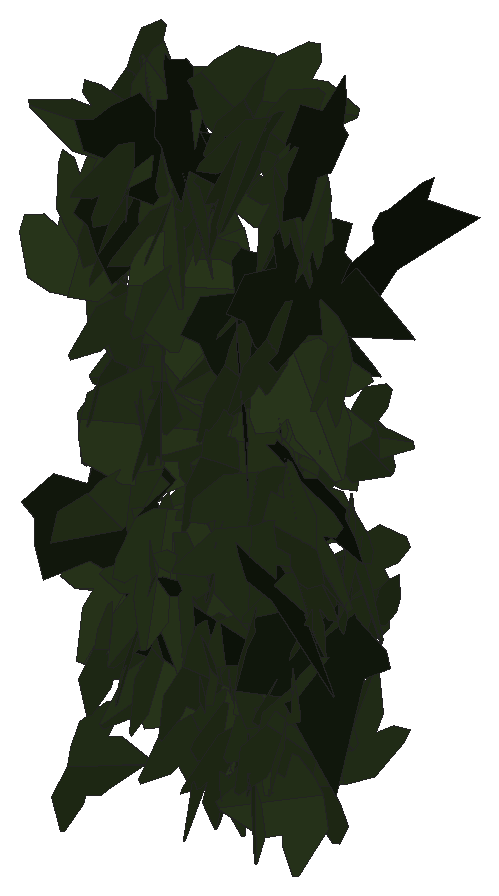
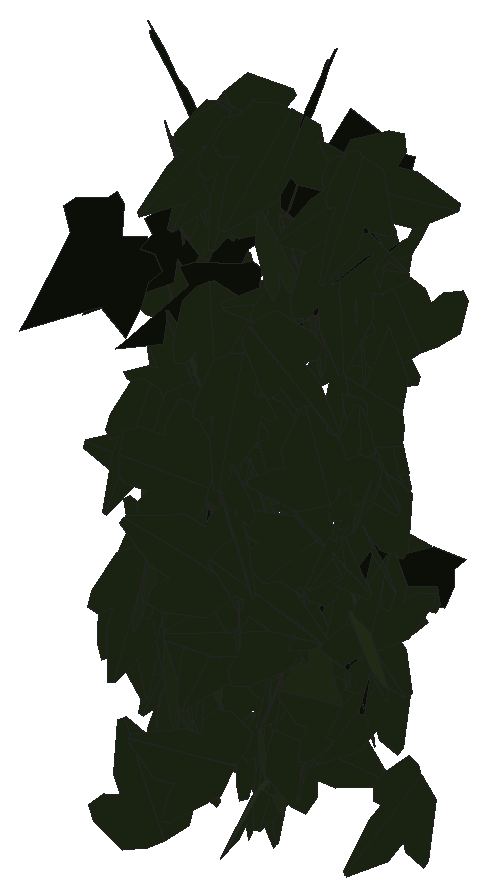
# SketchUp Ruby script. Lengths in inches.
U = 1.inch
M = Sketchup.active_model
def pt(a) = Geom::Point3d.new(a.map { |v| v * U })
def face(e, loops, mat)
  f = e.add_face(loops[0].map { |a| pt(a) })
  loops[1..].each { |l| e.add_face(l.map { |a| pt(a) }).erase! }
  f.material = f.back_material = mat if mat
  f
end
# faces: each face lists its corners as indices into pts; further lists are holes
def faces(e, pts, list, mat = nil) = list.each { |f| face(e, (f[0].is_a?(Array) ? f : [f]).map { |l| l.map { |i| pts[i] } }, mat) }
# xy, xz, yz: faces in a plane at the given z, y or x. An outline is a flat list of corners, or four numbers for a rectangle; further outlines are holes
def ring(l) = l.size == 4 ? [[l[0], l[1]], [l[2], l[1]], [l[2], l[3]], [l[0], l[3]]] : l.each_slice(2).to_a
def flat(e, list, mat, &to3) = list.each { |f| face(e, (f[0].is_a?(Array) ? f : [f]).map { |l| ring(l).map { |u, v| to3.(u, v) } }, mat) }
def xy(e, z, list, mat = nil) = flat(e, list, mat) { |x, y| [x, y, z] }
def xz(e, y, list, mat = nil) = flat(e, list, mat) { |x, z| [x, y, z] }
def yz(e, x, list, mat = nil) = flat(e, list, mat) { |y, z| [x, y, z] }
def lines(e, pts, list) = list.each { |a, b| e.add_line(pt(pts[a]), pt(pts[b])) }
# prism: a flat outline (further loops are holes) pulled along v
def prism(e, loops, v, mat = nil)
  f = face(e, loops, mat); d = Geom::Vector3d.new(v.map { |x| x * U })
  f.pushpull(f.normal.samedirection?(d) ? d.length : -d.length)
end
def box(e, o, s, mat = nil) = prism(e, [[o, [o[0] + s[0], o[1], o[2]], [o[0] + s[0], o[1] + s[1], o[2]], [o[0], o[1] + s[1], o[2]]]], [0, 0, s[2]], mat)
def at(x, y, z, deg = 0) = Geom::Transformation.translation(pt([x, y, z])) * Geom::Transformation.rotation(ORIGIN, Z_AXIS, deg.degrees)
def axes(o, x, y, z) = Geom::Transformation.new([*x, 0, *y, 0, *z, 0, *pt(o).to_a, 1])
def part(name) = M.definitions.add(name)
# library, detail: a bought-in or finely detailed component or shape, given as its bounding box
def library(name, o, s) = part(name).tap { |d| box(d.entities, o, s) }
def detail(e, o, s) = box(e.add_group.entities, o, s)
def put(e, d, t, mat = nil) = e.add_instance(d, t).tap { |i| i.material = mat if mat }
def group(e, t, mat = nil) = e.add_group.tap { |g| g.transformation = t; g.material = mat if mat }.entities
root = M.entities
M.materials.add("efeu1").color = [18, 25, 13]
M.materials.add("efeu2").color = [43, 57, 29]
c1 = part("ivyleaf_10")
p = [[0,0.5,-0.03],[-0.0625,2.02,-0.43],[-0.19,2.01,-0.46],[-0.54,1.05,-0.29],[-0.52,0.625,-0.18],[-0.83,0.76,-0.28],
  [-1.16,0.64,-0.33],[-1.15,0.33,-0.24],[-0.77,-0.39,0.02],[-0.3,-0.51,0.16],[0.04,-0.48,0.23],[-0.02,2.01,-0.4375],
  [-0.06,2.01,-0.43],[0.04,-0.49,0.23],[0.67,-0.49,0.14],[1.38,0.36,-0.2],[1.375,0.51,-0.24],[0.81,0.65,-0.19],
  [0.62,0.59,-0.15],[0.6,1.09,-0.28],[0.5,1.23,-0.31]]
faces(c1.entities,p,[[0,1,2,3,4,5,6,7,8,9,10],[11,12,0,13,14,15,16,17,18,19,20]],"efeu2")
c2 = part("ivyleaf_9")
p = [[1.54,2.16,1.25],[1.36,2.04,1.19],[-0.21,0.99,0.68],[-0.71,1.11,0.82],[-0.85,0.86,0.67],[-0.8,0.17,0.21],
  [-0.9,-0.01,0.1],[-0.67,-0.16,-0.02],[-0.08,-0.08,-0.05],[-0.03,-0.6,-0.4],[0.65,-0.88,-0.66],[0.83,-0.6,-0.49],
  [1.29,-0.42,-0.43],[1.8125,-0.07,-0.26],[1.21,0.44,0.15]]
faces(c2.entities,p,[[0,1,2,3,4,5,6,7,8,9,10,11,12,13,14]],"efeu1")
put(root,c1,axes([17.64,224.54,212.18],[0.2615,0.37788,-0.19704],[0.11551,0.15967,0.45952],[0.41021,-0.28585,-0.00379]))
put(root,c1,axes([17.67,225.08,210.66],[-0.06959,-0.33909,-0.3608],[0.20664,0.31121,-0.33234],[0.44995,-0.19537,0.09683]))
put(root,c1,axes([18.18,224.62,213.66],[-0.00757,0.03788,-0.49851],[-0.49654,0.0575,0.01191],[0.05823,0.49524,0.03675]))
put(root,c1,axes([17.86,224.87,209.08],[0.13792,0.47951,-0.03238],[-0.01347,0.03753,0.49841],[0.48041,-0.13661,0.02327]))
put(root,c1,axes([17.9,224.31,212.84],[0.04507,0.18765,-0.46125],[-0.0477,0.46264,0.18355],[0.49567,0.02745,0.0596]))
put(root,c1,axes([17.85,225.125,214.01],[-0.01418,-0.36054,-0.34613],[0.03369,0.3448,-0.36053],[0.49866,-0.03355,0.01451]))
put(root,c1,axes([17.9,225.35,213.2],[-0.1867,-0.46323,-0.0237],[0.00829,0.02221,-0.49944],[0.46376,-0.18688,-0.00061]))
put(root,c1,axes([17.83,224.4,207.17],[-0.04942,-0.21754,-0.44748],[0.10686,0.43454,-0.22305],[0.48594,-0.11768,0.00354]))
put(root,c1,axes([17.92,224.92,211.2],[-0.00617,-0.38233,-0.32216],[0.02352,0.32161,-0.38212],[0.49941,-0.01988,0.01402]))
put(root,c1,axes([18.3,224.91,211.08],[-0.17671,0.01361,0.46753],[-0.46773,-0.00286,-0.1767],[-0.00213,-0.49981,0.01374]))
put(root,c1,axes([17.75,225.18,211.18],[-0.20677,0.25144,-0.3795],[0.21731,-0.31174,-0.32495],[-0.40003,-0.29932,0.01963]))
put(root,c1,axes([17.87,225.59,210.96],[0.41138,0.26596,-0.10014],[0.08042,0.06005,0.48982],[0.27257,-0.41912,0.00663]))
put(root,c1,axes([17.71,225.07,208.91],[0.15502,-0.28412,-0.38111],[0.25032,-0.29199,0.3195],[-0.40411,-0.28986,0.05172]))
put(root,c1,axes([17.6,224.98,211.71],[-0.009,-0.05461,0.49693],[0.49966,-0.01693,0.00719],[0.01604,0.49672,0.05487]))
put(root,c2,axes([17.74,224.67,209.85],[0.01818,-0.30174,-0.39827],[0.13086,0.3875,-0.28761],[0.48223,-0.09378,0.09306]))
put(root,c1,axes([18.375,225.36,210.3],[-0.15751,-0.00285,0.47453],[-0.47294,-0.04009,-0.15722],[0.03894,-0.49838,0.00994]))
put(root,c1,axes([17.93,224.59,209.79],[-0.26802,-0.31765,-0.27796],[0.18909,0.20402,-0.41548],[0.37737,-0.32783,0.01077]))
put(root,c1,axes([18.04,224.74,212.79],[0.14301,-0.45229,-0.15806],[0.00861,0.16735,-0.47108],[0.47904,0.13201,0.05565]))
put(root,c1,axes([18.01,224.57,208.37],[-0.05576,-0.22516,-0.44294],[0.12172,0.42595,-0.23184],[0.48174,-0.13369,0.00731]))
put(root,c1,axes([17.74,224.99,209.85],[0.17654,-0.18081,-0.43144],[0.35353,-0.25042,0.24961],[-0.30635,-0.39319,0.03942]))
put(root,c1,axes([18.12,225.3,208.45],[0.18317,-0.24827,0.39346],[-0.16256,0.36205,0.30413],[-0.43592,-0.23933,0.05192]))
put(root,c1,axes([18.18,224.78,209.125],[0.4167,0.1887,-0.20188],[-0.18238,-0.08662,-0.45742],[-0.2076,0.45485,-0.00336]))
put(root,c1,axes([18.1,225.01,213.71],[-0.01135,-0.02598,-0.4992],[0.10029,0.48905,-0.02773],[0.48971,-0.10075,-0.00589]))
put(root,c1,axes([18.21,224.6875,213.42],[-0.00699,-0.48951,0.10164],[-0.00529,-0.10158,-0.48955],[0.49992,-0.00792,-0.00376]))
put(root,c2,axes([17.97,224.84,212.95],[0.26335,-0.29587,-0.30514],[-0.06558,0.32638,-0.37306],[0.41994,0.23651,0.1331]))
put(root,c1,axes([18.34,225.4,208],[-0.08271,-0.24704,0.42677],[-0.13867,-0.40361,-0.26051],[0.47321,-0.16145,-0.00174]))
put(root,c1,axes([18.21,224.68,211.92],[-0.18902,-0.43193,-0.16645],[0.0723,0.15004,-0.47144],[0.45721,-0.20229,0.00574]))
put(root,c1,axes([18.45,225.67,212.3],[0.29862,-0.09169,-0.39041],[-0.36462,0.14058,-0.31191],[0.16697,0.47099,0.0171]))
put(root,c1,axes([17.98,224.65,210.61],[0.07656,0.02642,0.4934],[0.23997,0.43446,-0.06049],[-0.43192,0.24606,0.05384]))
put(root,c1,axes([18.26,224.75,208.76],[0.28808,-0.40856,0.00918],[0.0027,-0.00933,-0.49991],[0.40866,0.28808,-0.00317]))
put(root,c1,axes([18.39,225.13,212.92],[0.15823,-0.46021,-0.11477],[-0.02025,0.11433,-0.48633],[0.47387,0.15855,0.01754]))
put(root,c1,axes([18.35,224.85,208.25],[0.07269,-0.37831,-0.31875],[0.06106,0.32657,-0.37367],[0.49091,0.0154,0.09367]))
put(root,c1,axes([18.43,224.88,212.78],[0.02384,-0.49721,0.04705],[0.0081,-0.04671,-0.49775],[0.49937,0.02449,0.00583]))
put(root,c1,axes([18.47,224.72,209.29],[-0.00281,-0.06953,-0.49513],[-0.02373,0.4946,-0.06932],[0.49943,0.02311,-0.00607]))
put(root,c1,axes([18.11,225.64,210.22],[0.32577,0.15564,0.3459],[0.29949,0.17425,-0.36047],[-0.23276,0.44205,0.0203]))
put(root,c1,axes([18.61,224.71,213.53],[0.34857,-0.09713,0.34506],[-0.33231,0.09292,0.36185],[-0.13442,-0.48159,0.00022]))
put(root,c1,axes([18.61,224.8125,209.14],[-0.16539,-0.36754,0.29591],[-0.11529,-0.27258,-0.403],[0.45755,-0.20154,0.00541]))
put(root,c1,axes([18.77,225.79,209.82],[0.26204,0.02235,-0.42525],[-0.42583,0.01467,-0.26163],[0.00078,0.49929,0.02672]))
put(root,c1,axes([18.56,224.59,211.07],[0.1821,-0.41178,-0.21743],[-0.02812,0.22332,-0.44647],[0.46481,0.17483,0.05818]))
put(root,c1,axes([18.89,224.78,208.43],[-0.07457,0.08537,-0.48698],[-0.40707,0.26891,0.10948],[0.2806,0.4128,0.02939]))
put(root,c1,axes([18.64,225.09,213.11],[0.3578,-0.30703,-0.16647],[-0.12497,0.11,-0.47147],[0.32613,0.37899,0.00198]))
put(root,c2,axes([18.17,224.59,213.44],[0.17994,0.00908,0.46641],[0.46649,-0.00108,-0.17996],[-0.00226,0.49992,-0.00886]))
put(root,c1,axes([18.57,224.71,209.62],[0.16219,0.45037,-0.14443],[-0.0584,-0.13245,-0.47859],[-0.46934,0.17212,0.00964]))
put(root,c1,axes([18.65,225.32,207.62],[-0.43569,0.11451,0.21693],[0.20765,-0.06322,0.45043],[0.13058,0.48259,0.00753]))
put(root,c1,axes([18.87,224.85,208.44],[0.10057,-0.0306,-0.48882],[-0.0991,0.48743,-0.05091],[0.47965,0.10712,0.09198]))
put(root,c2,axes([18.35,224.74,208.71],[0.22121,0.1206,-0.43188],[0.35154,0.25232,0.25052],[0.27837,-0.41448,0.02684]))
put(root,c1,axes([18.54,224.77,213.14],[0.37885,-0.18247,0.27052],[0.26742,-0.06391,-0.41761],[0.18698,0.46111,0.04917]))
put(root,c1,axes([18.71,224.8,212.35],[-0.18406,-0.38631,-0.25862],[0.16046,0.20826,-0.4253],[0.43632,-0.23956,0.04731]))
put(root,c1,axes([19.01,225.35,209.6],[0.34956,0.00602,0.35745],[-0.35547,0.05909,0.34663],[-0.03807,-0.49646,0.04559]))
put(root,c1,axes([18.79,225.2,213.23],[0.1265,-0.44392,0.19219],[0.05226,-0.18495,-0.46159],[0.4809,0.13687,-0.00039]))
put(root,c1,axes([19.1,225.02,208.37],[-0.40068,-0.01049,0.2989],[-0.29853,-0.01653,-0.40076],[0.01829,-0.49962,0.00698]))
put(root,c1,axes([18.63,224.7,209.39],[0.43192,-0.11056,0.22632],[0.22546,-0.0306,-0.44523],[0.1123,0.48666,0.02341]))
put(root,c1,axes([18.78,225.16,214.21],[-0.26561,-0.32596,-0.27056],[0.16918,0.21115,-0.42047],[0.38837,-0.31491,-0.00187]))
put(root,c1,axes([18.99,225.67,210.57],[0.31068,-0.25282,-0.29926],[-0.19872,0.22745,-0.39847],[0.33762,0.36653,0.04085]))
put(root,c1,axes([18.61,224.95,208.16],[0.39618,0.16741,0.25498],[0.22652,0.11843,-0.42972],[-0.20427,0.45601,0.01799]))
put(root,c1,axes([18.5625,224.61,212.3125],[-0.0135,-0.0784,-0.49363],[0.44217,0.22836,-0.04836],[0.23304,-0.43784,0.06316]))
put(root,c1,axes([18.88,224.8,207.73],[-0.19827,-0.40639,-0.21339],[0.09689,0.19016,-0.45216],[0.44867,-0.22065,0.00335]))
put(root,c2,axes([18.9,224.38,214.39],[0.26883,-0.15755,-0.39104],[-0.3176,0.22931,-0.31073],[0.27724,0.41545,0.02322]))
put(root,c1,axes([18.96,225.5,211.67],[-0.12469,-0.44761,-0.18465],[0.05343,0.17679,-0.46464],[0.48125,-0.1356,0.00375]))
put(root,c1,axes([18.96,225.09,207.28],[0.22271,-0.13905,-0.42552],[0.00503,0.47602,-0.15292],[0.44763,0.06383,0.21343]))
put(root,c1,axes([18.75,225.26,208.99],[0.02995,-0.08089,0.4925],[0.25836,0.42465,0.05404],[-0.42703,0.25125,0.06724]))
put(root,c1,axes([19.03,224.49,208.53],[-0.02806,-0.32135,-0.38203],[0.04211,0.37974,-0.32252],[0.49743,-0.05027,0.00575]))
put(root,c1,axes([19.06,225.32,211.47],[-0.04127,0.0057,-0.49826],[-0.12243,-0.48476,0.0046],[-0.48302,0.12238,0.04141]))
put(root,c1,axes([19,224.5,213.62],[-0.2848,0.41096,0.00067],[-0.00041,0.00053,-0.5],[-0.41096,-0.2848,0.00004]))
put(root,c1,axes([18.95,225.02,207.61],[0.18206,-0.3612,0.29392],[0.13835,-0.25938,-0.40445],[0.44465,0.2286,0.00551]))
put(root,c1,axes([19.11,225.02,207.58],[0.04931,-0.49739,-0.01299],[-0.00089,0.01296,-0.49983],[0.49756,0.04931,0.00039]))
put(root,c1,axes([19.05,225.19,211.21],[0.49808,-0.03349,-0.02821],[-0.02746,0.01204,-0.4991],[0.03411,0.49873,0.01015]))
put(root,c1,axes([18.92,225.91,207.82],[0.14371,0.17618,-0.44532],[0.27391,0.35114,0.22731],[0.39284,-0.30929,0.00441]))
put(root,c1,axes([19.12,225.23,214.02],[-0.11242,-0.42007,-0.24678],[0.06639,0.23769,-0.43485],[0.48265,-0.13054,0.00233]))
put(root,c1,axes([19.36,225.12,209.625],[-0.23062,0.18756,0.40204],[-0.34545,0.20837,-0.29537],[-0.27835,-0.41401,0.03348]))
put(root,c1,axes([19.14,224.92,210.16],[0.29836,-0.39089,0.0905],[0.06199,-0.06651,-0.49166],[0.39641,0.30461,0.00878]))
put(root,c1,axes([19,225.84,209.77],[-0.09889,-0.32395,0.3678],[0.21446,0.30878,0.32964],[-0.44071,0.22296,0.07788]))
put(root,c1,axes([19.68,224.97,210.52],[-0.08826,-0.03157,0.49113],[-0.47837,-0.11173,-0.09315],[0.11563,-0.48633,-0.01048]))
put(root,c1,axes([19.36,224.32,210.91],[0.0193,-0.29949,-0.39992],[0.01876,0.40037,-0.29892],[0.49928,-0.00347,0.02669]))
put(root,c1,axes([19.34,224.8125,213.81],[0.19916,-0.45166,0.07962],[0.02181,-0.07737,-0.4935],[0.45811,0.20004,-0.01111]))
put(root,c1,axes([19.5,225.34,211.1],[-0.47127,-0.06799,0.15258],[-0.14825,-0.0402,-0.47582],[0.07697,-0.49372,0.01773]))
put(root,c1,axes([19.41,225.34,212.2],[-0.0938,-0.48863,-0.04944],[0.00668,0.04906,-0.49754],[0.49108,-0.094,-0.00267]))
put(root,c1,axes([19.3,225.4375,214.09],[-0.02435,-0.24474,-0.43533],[0.19696,0.39581,-0.23354],[0.45893,-0.18285,0.07714]))
put(root,c1,axes([19.78,225.17,213.3],[0.06918,0.05139,-0.49252],[-0.49302,0.05364,-0.06366],[0.0463,0.49445,0.0581]))
put(root,c1,axes([19.5,224.87,214.03],[0.00975,-0.482,0.13259],[-0.01053,-0.13278,-0.48193],[0.49979,0.0066,-0.01274]))
put(root,c1,axes([19.39,225.08,208.875],[-0.32792,-0.3004,-0.22854],[0.16211,0.16132,-0.44463],[0.34087,-0.3657,-0.0084]))
put(root,c1,axes([19.48,224.5,211.78],[-0.00525,-0.34804,-0.35894],[0.02788,0.3582,-0.34773],[0.49919,-0.02367,0.01564]))
put(root,c1,axes([19.14,225.26,209.98],[0.09245,0.06472,0.4871],[0.3698,0.31722,-0.11233],[-0.32357,0.38103,0.01079]))
put(root,c1,axes([19.47,225.12,213.97],[-0.14401,-0.35418,-0.32221],[0.11517,0.30097,-0.3823],[0.46476,-0.18433,-0.0051]))
put(root,c1,axes([19.72,224.46,208.65],[-0.00398,-0.0129,0.49982],[-0.30944,0.39267,0.00767],[-0.39272,-0.30927,-0.01111]))
put(root,c2,axes([19.26,224.9375,212.26],[0.13956,-0.14688,-0.45711],[0.15377,0.46463,-0.10235],[0.45484,-0.11201,0.17486]))
put(root,c1,axes([19.65,224.62,210.54],[-0.22268,-0.44581,0.04087],[-0.01627,-0.03756,-0.49832],[0.44738,-0.22326,0.00222]))
put(root,c1,axes([19.66,224.57,210.01],[-0.29602,-0.40285,-0.00924],[0.00734,0.00607,-0.49991],[0.40289,-0.2961,0.00232]))
put(root,c1,axes([19.48,224.93,207.64],[-0.11139,0.39312,-0.28818],[0.082,-0.27628,-0.40859],[-0.48049,-0.13828,-0.00292]))
put(root,c2,axes([19.34,224.83,211.68],[0.01373,-0.02945,-0.49894],[0.47694,-0.14848,0.02189],[-0.14946,-0.47654,0.02402]))
put(root,c2,axes([19.83,224.86,210.82],[0.1669,-0.00507,-0.47129],[-0.46063,0.10413,-0.16425],[0.09982,0.48901,0.03009]))
put(root,c1,axes([19.59,226.01,207.06],[-0.1308,-0.47786,0.06737],[0.02066,0.06419,0.49543],[-0.48215,0.13239,0.00295]))
put(root,c1,axes([19.72,225.22,213.58],[0.06066,-0.43727,0.23476],[0.05507,-0.22912,-0.44099],[0.49324,0.07936,0.02037]))
put(root,c1,axes([20.07,224.75,207.4375],[0.22366,-0.06155,-0.44293],[-0.42761,0.1155,-0.23197],[0.13087,0.48257,-0.00097]))
put(root,c1,axes([19.67,225.58,208.49],[0.17487,-0.40721,0.23152],[0.16765,-0.17635,-0.4368],[0.43739,0.23039,0.07486]))
put(root,c1,axes([19.44,225.72,210.57],[-0.05154,-0.14036,0.47712],[0.4402,0.21036,0.10944],[-0.23145,0.43133,0.10189]))
put(root,c1,axes([19.77,225,213.6],[-0.16491,0.47179,0.01478],[-0.00673,0.0133,-0.49978],[-0.47197,-0.16504,0.00196]))
put(root,c1,axes([20.16,225.03,207.47],[-0.1996,0.0465,0.45607],[-0.45079,0.07052,-0.20448],[-0.08334,-0.49281,0.01377]))
put(root,c1,axes([19.77,224.9,208.4],[0.21095,-0.40624,0.20118],[0.07945,-0.18533,-0.45754],[0.44631,0.225,-0.01364]))
put(root,c1,axes([19.84,225.27,207.82],[0.06131,-0.46586,0.17093],[0.01997,-0.16977,-0.46987],[0.49582,0.06445,-0.00221]))
put(root,c1,axes([19.89,224.58,212.14],[-0.0473,-0.38855,-0.31112],[0.02292,0.31049,-0.39124],[0.49723,-0.05127,-0.01156]))
put(root,c1,axes([19.72,224.82,208.48],[0.43307,-0.18471,0.16833],[0.15796,-0.05865,-0.47075],[0.19365,0.46092,0.00756]))
put(root,c1,axes([19.95,225.13,209.45],[-0.17221,-0.46935,-0.0076],[0.0034,0.00685,-0.49994],[0.4694,-0.17224,0.00083]))
put(root,c1,axes([19.83,224.82,208.17],[-0.3375,-0.28229,-0.2375],[0.17427,0.16172,-0.43986],[0.32515,-0.37968,-0.01077]))
put(root,c1,axes([19.9,225.75,209.38],[-0.194,-0.42095,-0.18753],[0.09627,0.16196,-0.46314],[0.45066,-0.2158,0.01821]))
put(root,c1,axes([19.77,225.15,211.07],[0.48676,0.02274,-0.11203],[0.1111,0.02116,0.48704],[0.02689,-0.49903,0.01554]))
put(root,c2,axes([20.05,224.875,210.66],[0.30221,0.11221,-0.3822],[-0.37558,-0.07957,-0.32033],[-0.13271,0.48071,0.03619]))
put(root,c1,axes([20.29,224.59,210.26],[-0.06083,0.00059,0.49629],[-0.49427,0.04492,-0.06063],[-0.04466,-0.49798,-0.00488]))
put(root,c2,axes([19.61,224.85,209.67],[0.28634,-0.38228,0.14788],[0.10033,-0.10953,-0.47743],[0.39742,0.30309,0.01398]))
put(root,c1,axes([19.95,224.91,209.75],[-0.42684,0.2604,-0.00199],[0.00123,-0.00181,-0.5],[-0.2604,-0.42684,0.0009]))
put(root,c1,axes([19.99,225.36,209.27],[0.08227,-0.47627,-0.12806],[-0.00781,0.12856,-0.48313],[0.49312,0.08149,0.01371]))
put(root,c1,axes([19.73,225.22,211.35],[0.24572,-0.26095,-0.34861],[0.24379,-0.24923,0.3584],[-0.36081,-0.34611,0.00475]))
put(root,c1,axes([20.02,225.06,213.49],[0.38708,-0.30833,-0.07143],[-0.05003,0.05182,-0.49479],[0.31252,0.39019,0.00926]))
put(root,c2,axes([19.79,224.875,212.74],[0.15504,-0.12751,-0.45794],[-0.00702,0.48101,-0.13631],[0.4753,0.0487,0.14736]))
put(root,c1,axes([19.97,224.61,208.16],[-0.16759,-0.33125,-0.33495],[0.14453,0.30221,-0.37119],[0.44836,-0.22123,-0.00554]))
put(root,c2,axes([20.33,224.69,214.03],[-0.12317,0.27897,0.39624],[-0.16782,0.35899,-0.3049],[-0.45461,-0.2081,0.0052]))
put(root,c1,axes([19.89,224.91,210.28],[-0.35779,0.15912,-0.31092],[0.28462,-0.12516,-0.39157],[-0.20244,-0.45718,-0.00101]))
put(root,c1,axes([20.16,225.6875,209.03],[-0.00461,-0.49931,0.02582],[0.0013,-0.02583,-0.49933],[0.49998,-0.00453,0.00154]))
put(root,c1,axes([20.12,225.47,210.94],[-0.03917,-0.38343,-0.31851],[0.06593,0.3127,-0.38454],[0.49408,-0.07213,0.02606]))
put(root,c1,axes([20.08,224.78,208.46],[-0.16117,-0.36319,-0.30351],[0.13688,0.27116,-0.39716],[0.45309,-0.21111,0.01202]))
put(root,c1,axes([19.91,225.73,209.61],[-0.20887,0.24074,-0.38525],[0.25988,-0.28446,-0.31866],[-0.37261,-0.33335,-0.0063]))
put(root,c1,axes([20.28,224.95,212.1],[0.37875,-0.23785,-0.22355],[-0.18553,0.12487,-0.4472],[0.26856,0.42171,0.00633]))
put(root,c2,axes([20.04,225.04,208.99],[-0.07616,-0.45581,-0.1909],[0.02582,0.18922,-0.46209],[0.49349,-0.08024,-0.00528]))
put(root,c1,axes([20.34,225.11,209.47],[0.21972,-0.19614,0.40405],[-0.30921,0.26017,0.29444],[-0.32575,-0.37926,-0.00697]))
put(root,c1,axes([19.98,224.875,211.73],[0.40002,0.18182,0.2386],[0.21483,0.10394,-0.43937],[-0.20937,0.45403,0.00503]))
put(root,c2,axes([20.24,225.71,212.82],[-0.08056,0.15733,-0.46771],[-0.19295,0.42614,0.17658],[0.45418,0.20894,-0.00795]))
